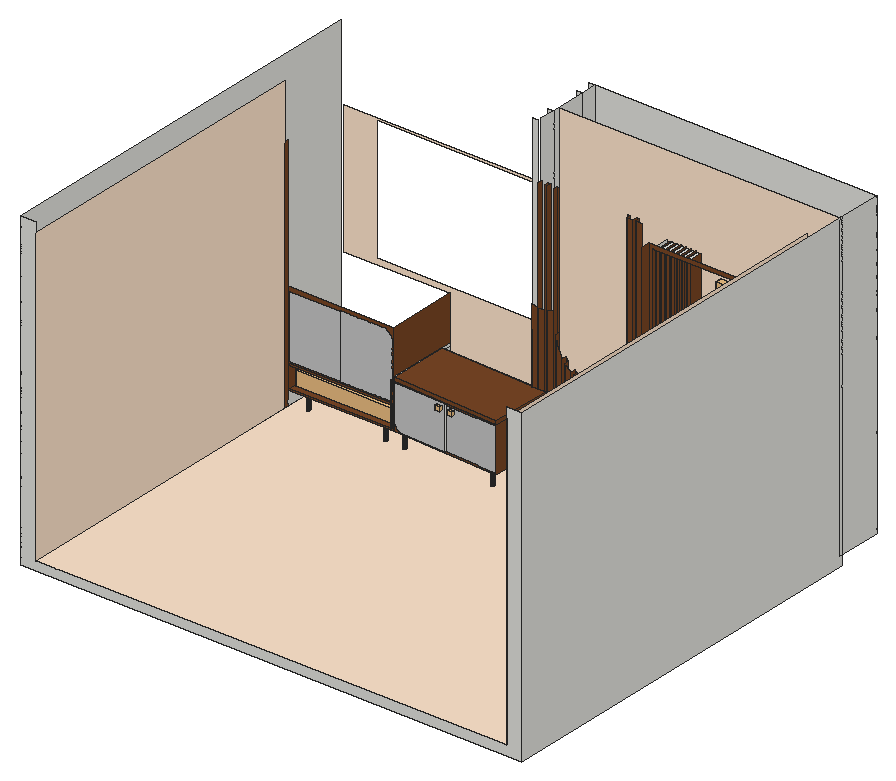
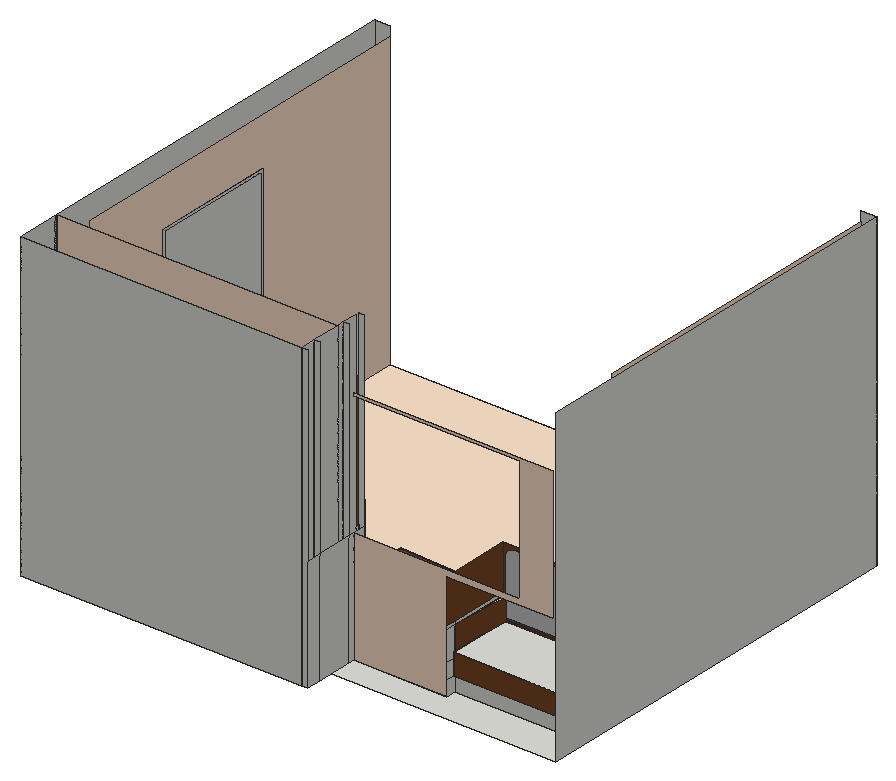
# SketchUp Ruby script. Lengths in inches.
U = 1.inch
M = Sketchup.active_model
def pt(a) = Geom::Point3d.new(a.map { |v| v * U })
def face(e, loops, mat)
  f = e.add_face(loops[0].map { |a| pt(a) })
  loops[1..].each { |l| e.add_face(l.map { |a| pt(a) }).erase! }
  f.material = f.back_material = mat if mat
  f
end
# faces: each face lists its corners as indices into pts; further lists are holes
def faces(e, pts, list, mat = nil) = list.each { |f| face(e, (f[0].is_a?(Array) ? f : [f]).map { |l| l.map { |i| pts[i] } }, mat) }
# xy, xz, yz: faces in a plane at the given z, y or x. An outline is a flat list of corners, or four numbers for a rectangle; further outlines are holes
def ring(l) = l.size == 4 ? [[l[0], l[1]], [l[2], l[1]], [l[2], l[3]], [l[0], l[3]]] : l.each_slice(2).to_a
def flat(e, list, mat, &to3) = list.each { |f| face(e, (f[0].is_a?(Array) ? f : [f]).map { |l| ring(l).map { |u, v| to3.(u, v) } }, mat) }
def xy(e, z, list, mat = nil) = flat(e, list, mat) { |x, y| [x, y, z] }
def xz(e, y, list, mat = nil) = flat(e, list, mat) { |x, z| [x, y, z] }
def yz(e, x, list, mat = nil) = flat(e, list, mat) { |y, z| [x, y, z] }
def lines(e, pts, list) = list.each { |a, b| e.add_line(pt(pts[a]), pt(pts[b])) }
# prism: a flat outline (further loops are holes) pulled along v
def prism(e, loops, v, mat = nil)
  f = face(e, loops, mat); d = Geom::Vector3d.new(v.map { |x| x * U })
  f.pushpull(f.normal.samedirection?(d) ? d.length : -d.length)
end
def box(e, o, s, mat = nil) = prism(e, [[o, [o[0] + s[0], o[1], o[2]], [o[0] + s[0], o[1] + s[1], o[2]], [o[0], o[1] + s[1], o[2]]]], [0, 0, s[2]], mat)
def at(x, y, z, deg = 0) = Geom::Transformation.translation(pt([x, y, z])) * Geom::Transformation.rotation(ORIGIN, Z_AXIS, deg.degrees)
def axes(o, x, y, z) = Geom::Transformation.new([*x, 0, *y, 0, *z, 0, *pt(o).to_a, 1])
def part(name) = M.definitions.add(name)
# library, detail: a bought-in or finely detailed component or shape, given as its bounding box
def library(name, o, s) = part(name).tap { |d| box(d.entities, o, s) }
def detail(e, o, s) = box(e.add_group.entities, o, s)
def put(e, d, t, mat = nil) = e.add_instance(d, t).tap { |i| i.material = mat if mat }
def group(e, t, mat = nil) = e.add_group.tap { |g| g.transformation = t; g.material = mat if mat }.entities
root = M.entities
M.materials.add("[Color C01]").color = [255, 229, 204]
M.materials.add("[Color M02]").color = [198, 198, 198]
M.materials.add("[Color M08]1").color = [30, 30, 30]
M.materials.add("[Metal Corrugated Shiny]").color = [193, 193, 193]
M.materials.add("[Wood Veneer 01]").color = [120, 70, 37]
c1 = library("Shoes",[47.68,11.3125,0],[16.97,82.95,11.27])
c2 = library("Group\#2",[0,0,0],[21.125,2.625,68.25])
c3 = library("Recessed spotlight",[0,0,0],[1.29,1.0625,0.73])
c4 = part("PHOTO+FRAME+WALL")
g1 = group(c4.entities,at(-24.55,1.0625,-0.57,-90))
xy(g1,0,[[0.83,0,1.18,49.09]])
xy(g1,0.57,[[0.83,0.57,1.0625,48.52]])
xy(g1,72.86,[[0.83,0.57,1.0625,48.52]])
xy(g1,73.43,[[0.83,0,1.18,49.09]])
xz(g1,0,[[0.83,0,1.18,73.43]])
xz(g1,0.57,[[0.83,0.57,1.0625,72.86]])
xz(g1,48.52,[[0.83,0.57,1.0625,72.86]])
xz(g1,49.09,[[0.83,0,1.18,73.43]])
yz(g1,0.83,[[[0,0,49.09,73.43],[0.57,0.57,48.52,72.86]]])
yz(g1,1.0625,[[0.57,0.57,48.52,72.86]])
yz(g1,1.18,[[0,0,49.09,73.43]])
c5 = library("Untitled (25)",[0,1.5,0.29],[5.35,2.09,5.32])
xy(root,0,[[0,0,198.4375,158.375]])
xy(root,3.75,[[84.82,147.02,84.82,147.26,87.07,147.17,87.07,147.02],[87.24,147.02,89.8,147.02,89.8,147.06,87.24,147.16],[90.74,147.02,90.74,148.71,89.8,148.71,89.8,147.06],[87.24,147.16,87.24,148.71,87.07,148.71,87.07,147.17],[87.07,147.17,87.07,147.26,84.82,147.26,84.82,152.4,47.85,152.4,47.85,148.71,84.82,147.26],
  [84.82,147.26,87.07,154.8125],[84.82,154.8125,87.07,169.1875],[87.07,157.4375,198.4375,175.3125],[84.82,169.1875,87.07,175.3125]])
xy(root,3.75,[[[6.1,0,192.34,0,192.34,148.71,191.3,148.71,191.3,146.15,188.74,146.15,188.74,148.71,187.8,148.71,187.8,146.15,185.24,146.15,185.24,148.71,184.3,148.71,184.3,150.65,128.3,150.65,128.3,147.02,125.74,147.02,125.74,148.71,124.8,148.71,124.8,147.02,122.24,147.02,122.24,148.71,121.3,148.71,121.3,147.02,118.74,147.02,118.74,148.71,117.8,148.71,117.8,147.02,115.24,147.02,115.24,148.71,114.3,148.71,114.3,147.02,111.74,147.02,111.74,148.71,110.8,148.71,110.8,147.02,108.24,147.02,108.24,148.71,107.3,148.71,107.3,147.02,104.74,147.02,104.74,148.71,103.8,148.71,103.8,147.02,101.24,147.02,101.24,148.71,100.3,148.71,100.3,147.02,97.74,147.02,97.74,148.71,96.8,148.71,96.8,147.02,94.24,147.02,94.24,148.71,93.3,148.71,93.3,147.02,90.74,147.02,89.8,147.06,89.8,147.02,87.24,147.02,87.24,147.16,87.07,147.17,87.07,147.02,84.82,147.02,84.82,147.26,47.85,148.71,6.1,148.71],[86.67,124.69,86.49,124.71,86.32,124.78,86.18,124.89,86.07,125.04,86,125.2,85.98,125.38,86,125.56,86.07,125.72,86.18,125.86,86.32,125.97,86.49,126.04,86.67,126.07,86.84,126.04,87.01,125.97,87.15,125.86,87.26,125.72,87.33,125.56,87.35,125.38,87.33,125.2,87.26,125.04,87.15,124.89,87.01,124.78,86.84,124.71],[50.69,126.11,50.52,126.13,50.35,126.2,50.21,126.31,50.1,126.45,50.03,126.62,50.01,126.79,50.03,126.97,50.1,127.14,50.21,127.28,50.35,127.39,50.52,127.46,50.69,127.48,50.87,127.46,51.04,127.39,51.18,127.28,51.29,127.14,51.36,126.97,51.38,126.79,51.36,126.62,51.29,126.45,51.18,126.31,51.04,126.2,50.87,126.13],[43,126.24,42.82,126.27,42.66,126.34,42.52,126.45,42.41,126.59,42.34,126.75,42.31,126.93,42.34,127.11,42.41,127.28,42.52,127.42,42.66,127.53,42.82,127.6,43,127.62,43.18,127.6,43.35,127.53,43.49,127.42,43.6,127.28,43.67,127.11,43.69,126.93,43.67,126.75,43.6,126.59,43.49,126.45,43.35,126.34,43.18,126.27],[12.5,126.24,12.32,126.27,12.16,126.34,12.02,126.45,11.91,126.59,11.84,126.75,11.81,126.93,11.84,127.11,11.91,127.28,12.02,127.42,12.16,127.53,12.32,127.6,12.5,127.62,12.68,127.6,12.85,127.53,12.99,127.42,13.1,127.28,13.17,127.11,13.19,126.93,13.17,126.75,13.1,126.59,12.99,126.45,12.85,126.34,12.68,126.27]]],"[Color C01]")
xy(root,5.125,[[129.68,152.25,131.15,158.375],[131.71,152.25,133.1875,158.375],[133.74,152.25,135.22,158.375],[135.77,152.25,137.25,158.375],[137.8,152.25,139.28,158.375],
  [139.83,152.25,141.3125,158.375],[141.87,152.25,143.35,158.375]])
xy(root,9.55,[[[89.8,123.06,47.85,124.71,47.85,148.71,84.82,147.26,90.74,147.02],[50.69,126.11,50.87,126.13,51.04,126.2,51.18,126.31,51.29,126.45,51.36,126.62,51.38,126.79,51.36,126.97,51.29,127.14,51.18,127.28,51.04,127.39,50.87,127.46,50.69,127.48,50.52,127.46,50.35,127.39,50.21,127.28,50.1,127.14,50.03,126.97,50.01,126.79,50.03,126.62,50.1,126.45,50.21,126.31,50.35,126.2,50.52,126.13],[86.67,124.69,86.84,124.71,87.01,124.78,87.15,124.89,87.26,125.04,87.33,125.2,87.35,125.38,87.33,125.56,87.26,125.72,87.15,125.86,87.01,125.97,86.84,126.04,86.67,126.07,86.49,126.04,86.32,125.97,86.18,125.86,86.07,125.72,86,125.56,85.98,125.38,86,125.2,86.07,125.04,86.18,124.89,86.32,124.78,86.49,124.71]],[[6.1,124.71,47.85,148.71],[12.5,126.24,12.68,126.27,12.85,126.34,12.99,126.45,13.1,126.59,13.17,126.75,13.19,126.93,13.17,127.11,13.1,127.28,12.99,127.42,12.85,127.53,12.68,127.6,12.5,127.62,12.32,127.6,12.16,127.53,12.02,127.42,11.91,127.28,11.84,127.11,11.81,126.93,11.84,126.75,11.91,126.59,12.02,126.45,12.16,126.34,12.32,126.27],[43,126.24,43.18,126.27,43.35,126.34,43.49,126.45,43.6,126.59,43.67,126.75,43.69,126.93,43.67,127.11,43.6,127.28,43.49,127.42,43.35,127.53,43.18,127.6,43,127.62,42.82,127.6,42.66,127.53,42.52,127.42,42.41,127.28,42.34,127.11,42.31,126.93,42.34,126.75,42.41,126.59,42.52,126.45,42.66,126.34,42.82,126.27]]])
xy(root,10.09,[[6.65,124.71,47.31,149.96]],"[Wood Veneer 01]")
xy(root,18.54,[[6.65,124.71,47.31,149.96]])
xy(root,27.41,[[89.8,123.06,47.85,124.71,47.85,148.71,84.82,147.26,90.74,147.02],[47.85,124.71,47.85,148.71,46.91,124.75]])
xy(root,28.66,[[89.8,123.06,90.74,147.02,84.82,147.26,47.85,148.71,47.85,124.71]],"[Wood Veneer 01]")
xy(root,91.72,[[131.71,152.25,133.1875,158.375],[133.74,152.25,135.22,158.375],[135.77,152.25,137.25,158.375],[137.8,152.25,139.28,158.375],[139.83,152.25,141.3125,158.375],
  [141.87,152.25,143.35,158.375]])
xz(root,0,[[0,0,198.4375,0,198.4375,123.75,192.34,123.75,192.34,3.75,6.1,3.75,6.1,123.75,0,123.75]])
xz(root,124.71,[[6.65,19.63,26.99,44.96],[26.99,19.63,47.31,19.63,47.31,41.08,47.28,41.58,47.18,42.08,47.01,42.5625,46.79,43.02,46.51,43.4375,46.17,43.82,45.79,44.15,45.37,44.4375,44.91,44.66,44.43,44.82,43.9375,44.92,43.43,44.96,26.99,44.96]],"[Color M02]")
xz(root,124.71,[[[6.1,9.55,47.85,19.09],[6.65,10.09,47.31,18.54]],[[6.1,19.09,47.85,46.25],[6.65,19.63,6.65,44.96,43.43,44.96,43.9375,44.92,44.43,44.82,44.91,44.66,45.37,44.4375,45.79,44.15,46.17,43.82,46.51,43.4375,46.79,43.02,47.01,42.5625,47.18,42.08,47.28,41.58,47.31,41.08,47.31,19.63]]],"[Wood Veneer 01]")
xz(root,146.15,[[185.24,3.75,187.8,101.64],[188.74,3.75,191.3,101.64]],"[Wood Veneer 01]")
xz(root,147.02,[[84.82,3.75,87.07,3.75,87.07,57.34,86.68,57.36,84.82,57.93],[87.24,3.75,89.8,3.75,89.8,57.32,89.5,57.25,87.24,57.34],[90.74,3.75,93.3,3.75,93.3,58.44,92.25,57.88,90.74,57.54],[94.24,3.75,96.8,3.75,96.8,42.4375,96.06,43.41,94.71,46.67,94.24,50.17],[97.74,3.75,100.3,3.75,100.3,39,98.21,40.61,97.74,41.21],
  [101.24,3.75,103.8,3.75,103.8,37.3,101.24,38.36],[104.74,3.75,107.3,3.75,107.3,36.71,104.74,37.04],[108.24,3.75,110.8,3.75,110.8,37.04,108.24,36.71],[111.74,3.75,114.3,3.75,114.3,38.36,111.74,37.3],[115.24,3.75,117.8,3.75,117.8,41.21,117.34,40.61,115.24,39],
  [118.74,3.75,121.3,3.75,121.3,50.17,120.84,46.67,119.49,43.41,118.74,42.4375],[122.24,3.75,124.8,101.64],[125.74,3.75,128.3,101.64]],"[Wood Veneer 01]")
xz(root,147.26,[[84.82,3.75,87.07,123.71]])
xz(root,148.71,[[6.1,3.75,47.85,9.55],[87.07,3.75,87.24,48.58]])
xz(root,148.71,[[89.8,3.75,90.74,101.64],[93.3,3.75,94.24,101.64],[96.8,3.75,97.74,3.75,97.74,41.21,96.8,42.4375],[100.3,3.75,101.24,3.75,101.24,38.36,101.01,38.46,100.3,39],[103.8,3.75,104.74,3.75,104.74,37.04,104.27,37.1,103.8,37.3],
  [107.3,3.75,108.24,3.75,108.24,36.71,107.77,36.64,107.3,36.71],[110.8,3.75,111.74,3.75,111.74,37.3,111.27,37.1,110.8,37.04],[114.3,3.75,115.24,3.75,115.24,39,114.54,38.46,114.3,38.36],[117.8,3.75,118.74,3.75,118.74,42.4375,117.8,41.21],[121.3,3.75,122.24,101.64],
  [124.8,3.75,125.74,101.64],[184.3,3.75,185.24,101.64],[187.8,3.75,188.74,101.64],[191.3,3.75,192.34,101.64]],"[Wood Veneer 01]")
xz(root,149.96,[[6.65,10.09,47.31,18.54]],"[Wood Veneer 01]")
xz(root,150.65,[[[128.3,3.75,184.3,93.09],[129.68,5.3125,182.93,91.66]]],"[Wood Veneer 01]")
xz(root,152.25,[[129.68,5.125,131.15,91.72],[131.71,5.125,133.1875,91.72],[133.74,5.125,135.22,91.72],[135.77,5.125,137.25,91.72],[137.8,5.125,139.28,91.72],
  [139.83,5.125,141.3125,91.72],[141.87,5.125,143.35,91.72]],"[Wood Veneer 01]")
xz(root,152.4,[[47.85,3.75,84.82,3.75,84.82,48.58,18.99,48.58,18.99,97.46,84.82,97.46,84.82,98.3,6.1,98.3,6.1,46.25,47.85,46.25]],"[Color C01]")
xz(root,154.8125,[[84.82,3.75,87.07,123.71]])
xz(root,157.4375,[[87.07,3.75,198.4375,123.71]],"[Color C01]")
xz(root,169.1875,[[84.82,3.75,87.07,123.71]])
xz(root,175.3125,[[84.82,3.75,87.07,123.71],[87.07,3.75,198.4375,123.71]])
yz(root,0,[[0,0,158.375,123.75]])
yz(root,6.1,[[124.71,3.75,148.71,9.55]])
yz(root,6.1,[[0,3.75,123.26,119.8125]],"[Color C01]")
yz(root,6.1,[[123.26,3.75,124.71,98.3]],"[Wood Veneer 01]")
yz(root,6.65,[[124.71,10.09,149.96,18.54]],"[Wood Veneer 01]")
yz(root,47.31,[[124.71,10.09,149.96,18.54]],"[Wood Veneer 01]")
yz(root,47.85,[[148.71,3.75,152.4,9.55],[124.71,9.55,152.4,9.55,152.4,15.96,148.71,15.96,124.71,19.09],[148.71,15.96,148.71,27.41,124.71,27.41,124.71,19.09],[148.71,15.96,152.4,27.41],[124.71,27.41,148.71,28.66],
  [148.71,27.41,152.4,28.66]])
yz(root,47.85,[[124.71,28.66,152.4,46.25]],"[Wood Veneer 01]")
yz(root,84.82,[[147.02,3.75,147.26,9.55],[147.26,3.75,152.4,48.58],[152.4,3.75,154.8125,48.58],[154.8125,3.75,169.1875,48.58],[169.1875,3.75,175.3125,48.58],
  [147.02,9.55,147.26,27.41],[147.02,27.41,147.26,48.58]])
yz(root,87.07,[[147.02,3.75,147.26,48.58],[147.26,3.75,148.71,48.58],[148.71,3.75,154.8125,123.71],[154.8125,3.75,157.4375,123.71],[157.4375,3.75,169.1875,123.71],
  [169.1875,3.75,175.3125,123.71]])
yz(root,87.24,[[147.02,3.75,148.71,101.64]],"[Wood Veneer 01]")
yz(root,89.8,[[147.02,3.75,148.71,101.64]],"[Wood Veneer 01]")
yz(root,90.74,[[147.02,3.75,148.71,101.64]],"[Wood Veneer 01]")
yz(root,93.3,[[147.02,3.75,148.71,101.64]],"[Wood Veneer 01]")
yz(root,94.24,[[147.02,3.75,148.71,50.17]],"[Wood Veneer 01]")
yz(root,96.8,[[147.02,3.75,148.71,42.4375]],"[Wood Veneer 01]")
yz(root,97.74,[[147.02,3.75,148.71,41.21]],"[Wood Veneer 01]")
yz(root,100.3,[[147.02,3.75,148.71,39]],"[Wood Veneer 01]")
yz(root,101.24,[[147.02,3.75,148.71,38.36]],"[Wood Veneer 01]")
yz(root,103.8,[[147.02,3.75,148.71,37.3]],"[Wood Veneer 01]")
yz(root,104.74,[[147.02,3.75,148.71,37.04]],"[Wood Veneer 01]")
yz(root,107.3,[[147.02,3.75,148.71,36.71]],"[Wood Veneer 01]")
yz(root,108.24,[[147.02,3.75,148.71,36.71]],"[Wood Veneer 01]")
yz(root,110.8,[[147.02,3.75,148.71,37.04]],"[Wood Veneer 01]")
yz(root,111.74,[[147.02,3.75,148.71,37.3]],"[Wood Veneer 01]")
yz(root,114.3,[[147.02,3.75,148.71,38.36]],"[Wood Veneer 01]")
yz(root,115.24,[[147.02,3.75,148.71,39]],"[Wood Veneer 01]")
yz(root,117.8,[[147.02,3.75,148.71,41.21]],"[Wood Veneer 01]")
yz(root,118.74,[[147.02,3.75,148.71,42.4375]],"[Wood Veneer 01]")
yz(root,121.3,[[147.02,3.75,148.71,50.17]],"[Wood Veneer 01]")
yz(root,122.24,[[147.02,3.75,148.71,101.64]],"[Wood Veneer 01]")
yz(root,124.8,[[147.02,3.75,148.71,101.64]],"[Wood Veneer 01]")
yz(root,125.74,[[147.02,3.75,148.71,101.64]],"[Wood Veneer 01]")
yz(root,128.3,[[147.02,3.75,150.65,93.09]],"[Wood Veneer 01]")
yz(root,129.68,[[152.25,5.125,158.375,5.3125],[152.25,5.3125,158.375,91.66]])
yz(root,129.68,[[150.65,5.3125,152.25,91.66]],"[Wood Veneer 01]")
yz(root,131.15,[[152.25,5.125,158.375,91.72]],"[Wood Veneer 01]")
yz(root,131.71,[[152.25,5.125,158.375,91.72]],"[Wood Veneer 01]")
yz(root,133.1875,[[152.25,5.125,158.375,91.72]],"[Wood Veneer 01]")
yz(root,133.74,[[152.25,5.125,158.375,91.72]],"[Wood Veneer 01]")
yz(root,135.22,[[152.25,5.125,158.375,91.72]],"[Wood Veneer 01]")
yz(root,135.77,[[152.25,5.125,158.375,91.72]],"[Wood Veneer 01]")
yz(root,137.25,[[152.25,5.125,158.375,91.72]],"[Wood Veneer 01]")
yz(root,137.8,[[152.25,5.125,158.375,91.72]],"[Wood Veneer 01]")
yz(root,139.28,[[152.25,5.125,158.375,91.72]],"[Wood Veneer 01]")
yz(root,139.83,[[152.25,5.125,158.375,91.72]],"[Wood Veneer 01]")
yz(root,141.3125,[[152.25,5.125,158.375,91.72]],"[Wood Veneer 01]")
yz(root,141.87,[[152.25,5.125,158.375,91.72]],"[Wood Veneer 01]")
yz(root,143.35,[[152.25,5.125,158.375,91.72]],"[Wood Veneer 01]")
yz(root,184.3,[[148.71,3.75,150.65,93.09]],"[Wood Veneer 01]")
yz(root,185.24,[[146.15,3.75,148.71,101.64]],"[Wood Veneer 01]")
yz(root,187.8,[[146.15,3.75,148.71,101.64]])
yz(root,188.74,[[146.15,3.75,148.71,101.64]],"[Wood Veneer 01]")
yz(root,191.3,[[146.15,3.75,148.71,101.64]])
yz(root,192.34,[[0,3.75,0,119.8125,148.71,119.8125,148.71,105.33,135.46,105.33,135.46,101.64,148.71,101.64,148.71,3.75]],"[Color C01]")
yz(root,198.4375,[[0,0,158.375,0,158.375,3.75,157.4375,3.75,157.4375,123.71,158.375,123.71,158.375,123.75,0,123.75],[157.4375,3.75,158.375,123.71],[158.375,3.75,175.3125,123.71]])
p = [[86.49,124.71,9.55],[86.32,124.78,9.55],[86.32,124.78,3.75],[86.49,124.71,3.75],[86.67,124.69,9.55],[86.67,124.69,3.75],
  [86.84,124.71,9.55],[86.84,124.71,3.75],[87.01,124.78,9.55],[87.01,124.78,3.75],[86.18,124.89,9.55],[86.18,124.89,3.75],
  [87.15,124.89,9.55],[87.15,124.89,3.75],[86.07,125.04,9.55],[86.07,125.04,3.75],[87.26,125.04,9.55],[87.26,125.04,3.75],
  [86,125.2,9.55],[86,125.2,3.75],[87.33,125.2,9.55],[87.33,125.2,3.75],[85.98,125.38,9.55],[85.98,125.38,3.75],
  [87.35,125.38,9.55],[87.35,125.38,3.75],[86,125.56,9.55],[86,125.56,3.75],[87.33,125.56,9.55],[87.33,125.56,3.75],
  [86.07,125.72,9.55],[86.07,125.72,3.75],[87.26,125.72,9.55],[87.26,125.72,3.75],[86.18,125.86,9.55],[86.18,125.86,3.75],
  [87.15,125.86,9.55],[87.15,125.86,3.75],[86.32,125.97,9.55],[86.32,125.97,3.75],[87.01,125.97,9.55],[87.01,125.97,3.75],
  [86.49,126.04,9.55],[86.49,126.04,3.75],[86.67,126.07,9.55],[86.67,126.07,3.75],[86.84,126.04,9.55],[86.84,126.04,3.75],
  [50.52,126.13,9.55],[50.35,126.2,9.55],[50.35,126.2,3.75],[50.52,126.13,3.75],[50.69,126.11,9.55],[50.69,126.11,3.75],
  [50.87,126.13,9.55],[50.87,126.13,3.75],[51.04,126.2,9.55],[51.04,126.2,3.75],[12.5,126.24,9.55],[12.32,126.27,9.55],
  [12.32,126.27,3.75],[12.5,126.24,3.75],[12.68,126.27,9.55],[12.68,126.27,3.75],[43,126.24,9.55],[42.82,126.27,9.55],
  [42.82,126.27,3.75],[43,126.24,3.75],[43.18,126.27,9.55],[43.18,126.27,3.75],[50.21,126.31,9.55],[50.21,126.31,3.75],
  [51.18,126.31,9.55],[51.18,126.31,3.75],[12.16,126.34,9.55],[12.02,126.45,9.55],[12.02,126.45,3.75],[12.16,126.34,3.75],
  [12.85,126.34,9.55],[12.85,126.34,3.75],[12.99,126.45,9.55],[12.99,126.45,3.75],[42.66,126.34,9.55],[42.52,126.45,9.55],
  [42.52,126.45,3.75],[42.66,126.34,3.75],[43.35,126.34,9.55],[43.35,126.34,3.75],[43.49,126.45,9.55],[43.49,126.45,3.75],
  [50.1,126.45,9.55],[50.1,126.45,3.75],[51.29,126.45,9.55],[51.29,126.45,3.75],[11.91,126.59,9.55],[11.91,126.59,3.75],
  [13.1,126.59,9.55],[13.1,126.59,3.75],[42.41,126.59,9.55],[42.41,126.59,3.75],[43.6,126.59,9.55],[43.6,126.59,3.75],
  [50.03,126.62,9.55],[50.03,126.62,3.75],[51.36,126.62,9.55],[51.36,126.62,3.75],[11.84,126.75,9.55],[11.84,126.75,3.75],
  [13.17,126.75,9.55],[13.17,126.75,3.75],[42.34,126.75,9.55],[42.34,126.75,3.75],[43.67,126.75,9.55],[43.67,126.75,3.75],
  [50.01,126.79,9.55],[50.01,126.79,3.75],[51.38,126.79,9.55],[51.38,126.79,3.75],[11.81,126.93,9.55],[11.81,126.93,3.75],
  [13.19,126.93,9.55],[13.19,126.93,3.75],[42.31,126.93,9.55],[42.31,126.93,3.75],[43.69,126.93,9.55],[43.69,126.93,3.75],
  [50.03,126.97,9.55],[50.03,126.97,3.75],[51.36,126.97,9.55],[51.36,126.97,3.75],[11.84,127.11,9.55],[11.84,127.11,3.75],
  [13.17,127.11,9.55],[13.17,127.11,3.75],[42.34,127.11,9.55],[42.34,127.11,3.75],[43.67,127.11,9.55],[43.67,127.11,3.75],
  [50.1,127.14,9.55],[50.1,127.14,3.75],[51.29,127.14,9.55],[51.29,127.14,3.75],[11.91,127.28,9.55],[11.91,127.28,3.75],
  [13.1,127.28,9.55],[13.1,127.28,3.75],[42.41,127.28,9.55],[42.41,127.28,3.75],[43.6,127.28,9.55],[43.6,127.28,3.75],
  [50.21,127.28,9.55],[50.21,127.28,3.75],[51.18,127.28,9.55],[51.18,127.28,3.75],[12.02,127.42,9.55],[12.02,127.42,3.75],
  [12.99,127.42,9.55],[12.99,127.42,3.75],[42.52,127.42,9.55],[42.52,127.42,3.75],[43.49,127.42,9.55],[43.49,127.42,3.75],
  [50.35,127.39,9.55],[50.35,127.39,3.75],[51.04,127.39,9.55],[51.04,127.39,3.75],[12.16,127.53,9.55],[12.16,127.53,3.75],
  [12.85,127.53,9.55],[12.85,127.53,3.75],[42.66,127.53,9.55],[42.66,127.53,3.75],[43.35,127.53,9.55],[43.35,127.53,3.75],
  [50.52,127.46,9.55],[50.52,127.46,3.75],[50.87,127.46,9.55],[50.87,127.46,3.75],[12.32,127.6,9.55],[12.32,127.6,3.75],
  [12.68,127.6,9.55],[12.68,127.6,3.75],[42.82,127.6,9.55],[42.82,127.6,3.75],[43.18,127.6,9.55],[43.18,127.6,3.75],
  [50.69,127.48,9.55],[50.69,127.48,3.75],[12.5,127.62,9.55],[12.5,127.62,3.75],[43,127.62,9.55],[43,127.62,3.75],
  [90.74,147.02,9.55],[84.82,147.26,9.55],[84.82,147.26,3.75],[87.07,147.17,3.75],[87.24,147.16,3.75],[89.8,147.06,3.75],
  [90.74,147.02,3.75],[47.85,148.71,3.75],[47.85,148.71,9.55],[89.8,123.06,9.55],[89.8,123.06,27.41],[47.85,124.71,27.41],
  [47.85,124.71,19.09],[47.85,124.71,9.55],[68.83,123.88,10.09],[51.7,124.56,10.09],[51.27,124.58,10.12],[50.85,124.59,10.21],
  [50.4375,124.61,10.35],[50.05,124.625,10.54],[49.6875,124.64,10.78],[49.36,124.65,11.0625],[49.08,124.66,11.39],[48.84,124.67,11.75],
  [48.65,124.68,12.14],[48.51,124.68,12.55],[48.42,124.6875,12.97],[48.4,124.6875,13.4],[48.4,124.6875,19.09],[48.4,124.6875,26.86],
  [68.83,123.88,26.86],[69.26,123.87,26.86],[89.26,123.08,26.86],[89.26,123.08,19.09],[89.26,123.08,10.09],[69.26,123.87,10.09],
  [90.74,147.02,27.41],[46.91,124.75,9.55],[46.91,124.75,27.41],[46.91,124.75,15.96],[69.26,123.87,19.09],[68.83,123.88,19.09],
  [47.85,148.71,27.41],[47.85,148.71,15.96],[47.85,124.71,28.66],[89.8,123.06,28.66],[90.74,147.02,28.66],[84.82,147.26,27.41],
  [84.82,147.26,28.66],[47.85,148.71,28.66]]
faces(root,p,[[0,1,2,3],[4,0,3,5],[6,4,5,7],[8,6,7,9],[1,10,11,2],[12,8,9,13],[10,14,15,11],[16,12,13,17],
  [14,18,19,15],[20,16,17,21],[18,22,23,19],[24,20,21,25],[22,26,27,23],[28,24,25,29],[26,30,31,27],[32,28,29,33],
  [30,34,35,31],[36,32,33,37],[34,38,39,35],[40,36,37,41],[38,42,43,39],[42,44,45,43],[44,46,47,45],[46,40,41,47],
  [48,49,50,51],[52,48,51,53],[54,52,53,55],[56,54,55,57],[58,59,60,61],[62,58,61,63],[64,65,66,67],[68,64,67,69],
  [49,70,71,50],[72,56,57,73],[74,75,76,77],[59,74,77,60],[78,62,63,79],[80,78,79,81],[82,83,84,85],[65,82,85,66],
  [86,68,69,87],[88,86,87,89],[70,90,91,71],[92,72,73,93],[75,94,95,76],[96,80,81,97],[83,98,99,84],[100,88,89,101],
  [90,102,103,91],[104,92,93,105],[94,106,107,95],[108,96,97,109],[98,110,111,99],[112,100,101,113],[102,114,115,103],[116,104,105,117],
  [106,118,119,107],[120,108,109,121],[110,122,123,111],[124,112,113,125],[114,126,127,115],[128,116,117,129],[118,130,131,119],[132,120,121,133],
  [122,134,135,123],[136,124,125,137],[126,138,139,127],[140,128,129,141],[130,142,143,131],[144,132,133,145],[134,146,147,135],[148,136,137,149],
  [138,150,151,139],[152,140,141,153],[142,154,155,143],[156,144,145,157],[146,158,159,147],[160,148,149,161],[150,162,163,151],[164,152,153,165],
  [154,166,167,155],[168,156,157,169],[158,170,171,159],[172,160,161,173],[162,174,175,163],[176,164,165,177],[166,178,179,167],[180,168,169,181],
  [170,182,183,171],[184,172,173,185],[174,186,187,175],[186,176,177,187],[178,188,189,179],[188,180,181,189],[182,190,191,183],[190,184,185,191]],"[Metal Corrugated Shiny]")
faces(root,p,[[192,193,194,195,196,197,198],[199,194,193,200],[206,227,232,223,222,233],[228,239,240,238],[239,234,241,240]])
faces(root,p,[[[201,202,203,204,205],[206,207,208,209,210,211,212,213,214,215,216,217,218,219,220,221,222,223,224,225,226,227]],[192,228,202,201],[229,205,204,203,230,231],[234,235,231,230],[236,203,202,237],[237,202,228,238]],"[Wood Veneer 01]")
faces(root,p,[[224,223,232,227,226,225],[220,219,218,217,216,215,214,213,212,211,210,209,208,207,206,233,222,221]],"[Color M02]")
detail(root,[151.26,157.5625,17.46],[21.13,0.8125,68.25])
put(root,c1,axes([1.51,150.91,10.09],[0,-0.3604,0],[0.47876,0,0],[0,0,0.48463]))
put(root,c2,at(151.375,154.8125,17.45))
put(root,c3,axes([65.75,124.01,24.28],[1.55,0,0],[0,0,1.55],[0,-1.55,0]),"[Color M08]1")
put(root,c3,axes([70.7,123.87,24.33],[1.55,0,0],[0,0,1.55],[0,-1.55,0]),"[Color M08]1")
put(root,c4,at(192.22,88.16,28.1875,90))
put(root,c5,axes([133.74,147.15,35.39],[1.42,0,0],[0,1.42,0],[0,0,1.42]))
